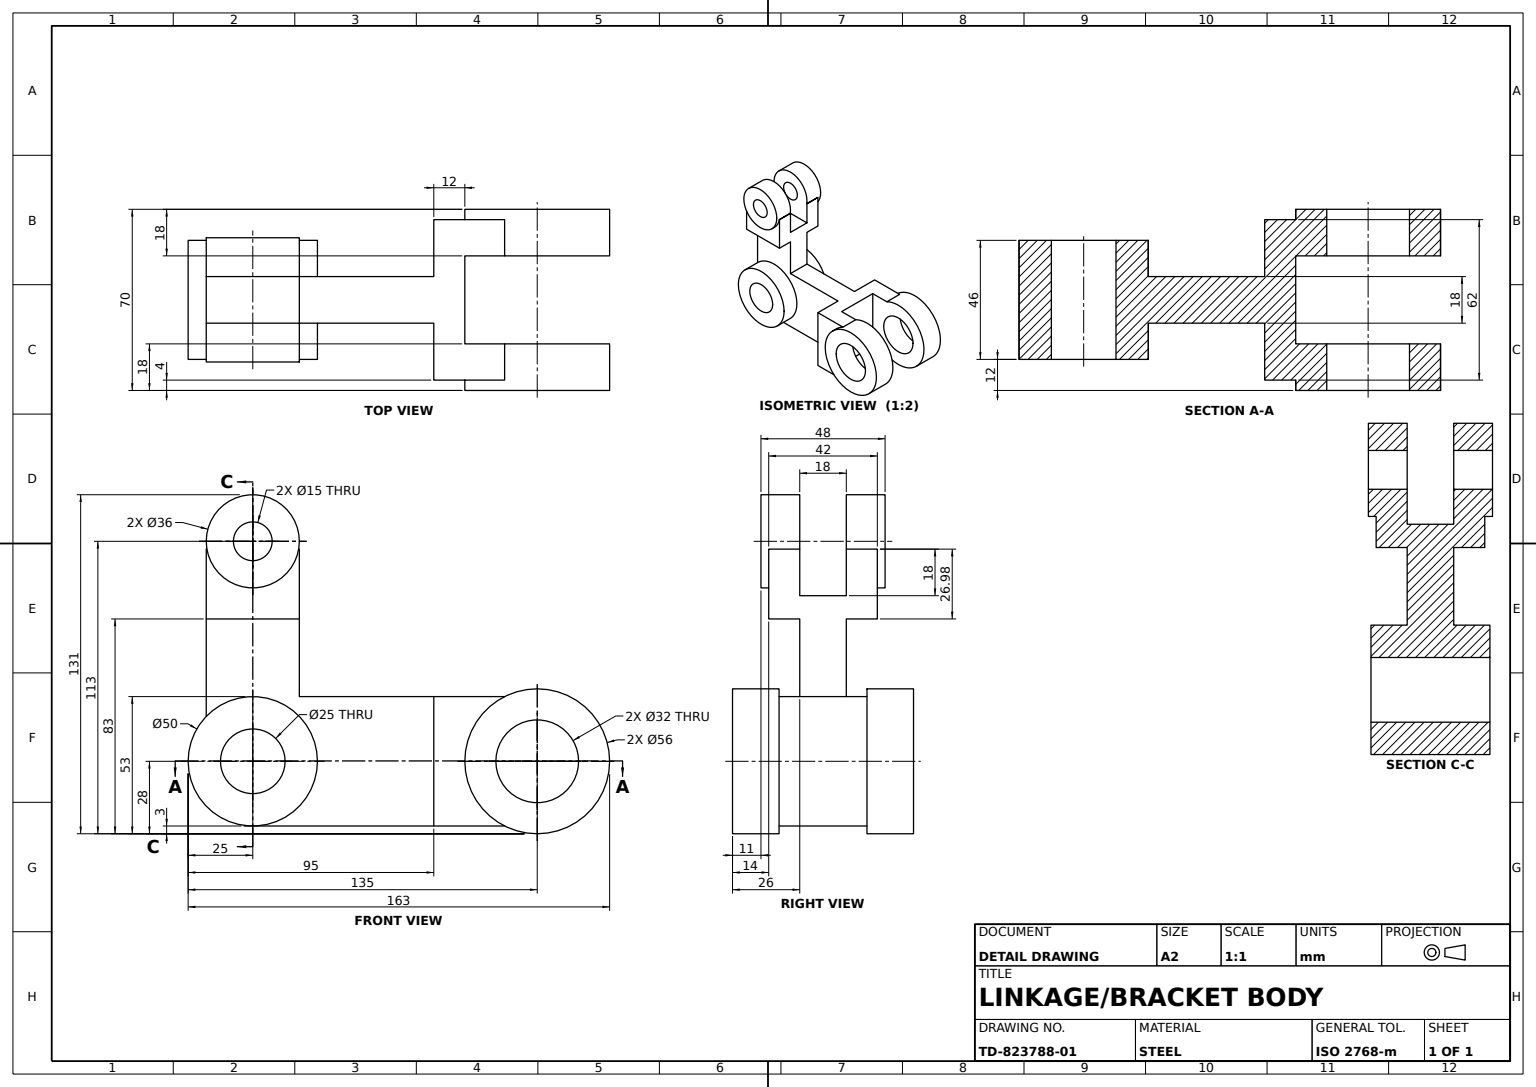
ISO-10303-21;
HEADER;
FILE_DESCRIPTION((''),'2;1');
FILE_NAME('','',(''),(''),'','','');
FILE_SCHEMA(('AUTOMOTIVE_DESIGN'));
ENDSEC;
DATA;
#1=APPLICATION_CONTEXT('');
#2=PRODUCT_CONTEXT('',#1,'mechanical');
#3=PRODUCT('','','',(#2));
#4=PRODUCT_DEFINITION_FORMATION('','',#3);
#5=PRODUCT_DEFINITION_CONTEXT('',#1,'design');
#6=PRODUCT_DEFINITION('','',#4,#5);
#7=PRODUCT_DEFINITION_SHAPE('','',#6);
#8=(LENGTH_UNIT()NAMED_UNIT(*)SI_UNIT(.MILLI.,.METRE.));
#9=(NAMED_UNIT(*)PLANE_ANGLE_UNIT()SI_UNIT($,.RADIAN.));
#10=(NAMED_UNIT(*)SI_UNIT($,.STERADIAN.)SOLID_ANGLE_UNIT());
#11=UNCERTAINTY_MEASURE_WITH_UNIT(LENGTH_MEASURE(1.E-05),#8,'distance_accuracy_value','');
#12=(GEOMETRIC_REPRESENTATION_CONTEXT(3)GLOBAL_UNCERTAINTY_ASSIGNED_CONTEXT((#11))GLOBAL_UNIT_ASSIGNED_CONTEXT((#8,#9,#10))REPRESENTATION_CONTEXT('',''));
#13=CARTESIAN_POINT('',(7.,110.,89.5));
#14=VERTEX_POINT('',#13);
#15=CARTESIAN_POINT('',(22.,110.,89.5));
#16=VERTEX_POINT('',#15);
#17=CARTESIAN_POINT('',(-5.,110.,89.5));
#18=DIRECTION('',(1.,0.,0.));
#19=VECTOR('',#18,1000.);
#20=LINE('',#17,#19);
#21=EDGE_CURVE('',#14,#16,#20,.T.);
#22=ORIENTED_EDGE('',*,*,#21,.F.);
#23=CARTESIAN_POINT('',(7.,110.,74.5));
#24=VERTEX_POINT('',#23);
#25=CARTESIAN_POINT('',(7.,110.,82.));
#26=DIRECTION('',(-1.,0.,0.));
#27=DIRECTION('',(0.,0.,1.));
#28=AXIS2_PLACEMENT_3D('',#25,#26,#27);
#29=CIRCLE('',#28,7.5);
#30=EDGE_CURVE('',#14,#24,#29,.T.);
#31=ORIENTED_EDGE('',*,*,#30,.T.);
#32=CARTESIAN_POINT('',(22.,110.,74.5));
#33=VERTEX_POINT('',#32);
#34=CARTESIAN_POINT('',(-5.,110.,74.5));
#35=LINE('',#34,#19);
#36=EDGE_CURVE('',#24,#33,#35,.T.);
#37=ORIENTED_EDGE('',*,*,#36,.T.);
#38=CARTESIAN_POINT('',(22.,110.,82.));
#39=AXIS2_PLACEMENT_3D('',#38,#26,#27);
#40=CIRCLE('',#39,7.5);
#41=EDGE_CURVE('',#16,#33,#40,.T.);
#42=ORIENTED_EDGE('',*,*,#41,.F.);
#43=EDGE_LOOP('',(#22,#31,#37,#42));
#44=FACE_OUTER_BOUND('',#43,.T.);
#45=CARTESIAN_POINT('',(-5.,110.,82.));
#46=DIRECTION('',(0.,0.,-1.));
#47=AXIS2_PLACEMENT_3D('',#45,#18,#46);
#48=CYLINDRICAL_SURFACE('',#47,7.5);
#49=ADVANCED_FACE('',(#44),#48,.F.);
#50=CARTESIAN_POINT('',(66.,25.,0.));
#51=VERTEX_POINT('',#50);
#52=CARTESIAN_POINT('',(66.,25.,-56.));
#53=VERTEX_POINT('',#52);
#54=CARTESIAN_POINT('',(66.,25.,-28.));
#55=AXIS2_PLACEMENT_3D('',#54,#18,#46);
#56=CIRCLE('',#55,28.);
#57=EDGE_CURVE('',#51,#53,#56,.T.);
#58=ORIENTED_EDGE('',*,*,#57,.T.);
#59=EDGE_CURVE('',#53,#51,#56,.T.);
#60=ORIENTED_EDGE('',*,*,#59,.T.);
#61=EDGE_LOOP('',(#58,#60));
#62=FACE_OUTER_BOUND('',#61,.T.);
#63=CARTESIAN_POINT('',(66.,25.,-44.));
#64=VERTEX_POINT('',#63);
#65=CARTESIAN_POINT('',(66.,25.,-12.));
#66=VERTEX_POINT('',#65);
#67=CIRCLE('',#55,16.);
#68=EDGE_CURVE('',#64,#66,#67,.T.);
#69=ORIENTED_EDGE('',*,*,#68,.F.);
#70=EDGE_CURVE('',#66,#64,#67,.T.);
#71=ORIENTED_EDGE('',*,*,#70,.F.);
#72=EDGE_LOOP('',(#69,#71));
#73=FACE_BOUND('',#72,.T.);
#74=PLANE('',#55);
#75=ADVANCED_FACE('',(#62,#73),#74,.T.);
#76=CARTESIAN_POINT('',(22.,80.,64.));
#77=VERTEX_POINT('',#76);
#78=CARTESIAN_POINT('',(10.,80.,64.));
#79=VERTEX_POINT('',#78);
#80=VECTOR('',#26,1000.);
#81=LINE('',#76,#80);
#82=EDGE_CURVE('',#77,#79,#81,.T.);
#83=ORIENTED_EDGE('',*,*,#82,.F.);
#84=CARTESIAN_POINT('',(22.,80.,100.));
#85=VERTEX_POINT('',#84);
#86=VECTOR('',#46,1000.);
#87=LINE('',#76,#86);
#88=EDGE_CURVE('',#85,#77,#87,.T.);
#89=ORIENTED_EDGE('',*,*,#88,.F.);
#90=CARTESIAN_POINT('',(10.,80.,100.));
#91=VERTEX_POINT('',#90);
#92=LINE('',#84,#80);
#93=EDGE_CURVE('',#85,#91,#92,.T.);
#94=ORIENTED_EDGE('',*,*,#93,.T.);
#95=LINE('',#78,#86);
#96=EDGE_CURVE('',#91,#79,#95,.T.);
#97=ORIENTED_EDGE('',*,*,#96,.T.);
#98=EDGE_LOOP('',(#83,#89,#94,#97));
#99=FACE_OUTER_BOUND('',#98,.T.);
#100=DIRECTION('',(0.,1.,0.));
#101=AXIS2_PLACEMENT_3D('',#76,#100,#27);
#102=PLANE('',#101);
#103=ADVANCED_FACE('',(#99),#102,.F.);
#104=CARTESIAN_POINT('',(40.,0.,85.354634));
#105=VERTEX_POINT('',#104);
#106=CARTESIAN_POINT('',(40.,0.226094,85.354634));
#107=VERTEX_POINT('',#106);
#108=VECTOR('',#100,1000.);
#109=LINE('',#104,#108);
#110=EDGE_CURVE('',#105,#107,#109,.T.);
#111=ORIENTED_EDGE('',*,*,#110,.F.);
#112=CARTESIAN_POINT('',(40.,0.,82.));
#113=VERTEX_POINT('',#112);
#114=LINE('',#104,#86);
#115=EDGE_CURVE('',#105,#113,#114,.T.);
#116=ORIENTED_EDGE('',*,*,#115,.T.);
#117=CARTESIAN_POINT('',(40.,25.,82.));
#118=AXIS2_PLACEMENT_3D('',#117,#26,#46);
#119=CIRCLE('',#118,25.);
#120=EDGE_CURVE('',#113,#107,#119,.T.);
#121=ORIENTED_EDGE('',*,*,#120,.T.);
#122=EDGE_LOOP('',(#111,#116,#121));
#123=FACE_OUTER_BOUND('',#122,.T.);
#124=CARTESIAN_POINT('',(40.,0.,71.244384));
#125=AXIS2_PLACEMENT_3D('',#124,#18,#46);
#126=PLANE('',#125);
#127=ADVANCED_FACE('',(#123),#126,.T.);
#128=CARTESIAN_POINT('',(40.,106.982899,100.));
#129=VERTEX_POINT('',#128);
#130=CARTESIAN_POINT('',(52.,106.982899,100.));
#131=VERTEX_POINT('',#130);
#132=CARTESIAN_POINT('',(0.,106.982899,100.));
#133=LINE('',#132,#19);
#134=EDGE_CURVE('',#129,#131,#133,.T.);
#135=ORIENTED_EDGE('',*,*,#134,.F.);
#136=CARTESIAN_POINT('',(40.,88.982899,100.));
#137=VERTEX_POINT('',#136);
#138=CARTESIAN_POINT('',(40.,0.,100.));
#139=LINE('',#138,#108);
#140=EDGE_CURVE('',#137,#129,#139,.T.);
#141=ORIENTED_EDGE('',*,*,#140,.F.);
#142=CARTESIAN_POINT('',(22.,88.982899,100.));
#143=VERTEX_POINT('',#142);
#144=LINE('',#142,#80);
#145=EDGE_CURVE('',#137,#143,#144,.T.);
#146=ORIENTED_EDGE('',*,*,#145,.T.);
#147=CARTESIAN_POINT('',(22.,106.982899,100.));
#148=VERTEX_POINT('',#147);
#149=CARTESIAN_POINT('',(22.,0.,100.));
#150=DIRECTION('',(0.,-1.,0.));
#151=VECTOR('',#150,1000.);
#152=LINE('',#149,#151);
#153=EDGE_CURVE('',#148,#143,#152,.T.);
#154=ORIENTED_EDGE('',*,*,#153,.F.);
#155=CARTESIAN_POINT('',(10.,106.982899,100.));
#156=VERTEX_POINT('',#155);
#157=EDGE_CURVE('',#156,#148,#133,.T.);
#158=ORIENTED_EDGE('',*,*,#157,.F.);
#159=CARTESIAN_POINT('',(10.,0.,100.));
#160=LINE('',#159,#108);
#161=EDGE_CURVE('',#91,#156,#160,.T.);
#162=ORIENTED_EDGE('',*,*,#161,.F.);
#163=ORIENTED_EDGE('',*,*,#93,.F.);
#164=CARTESIAN_POINT('',(22.,42.349352,100.));
#165=VERTEX_POINT('',#164);
#166=EDGE_CURVE('',#85,#165,#152,.T.);
#167=ORIENTED_EDGE('',*,*,#166,.T.);
#168=CARTESIAN_POINT('',(40.,42.349352,100.));
#169=VERTEX_POINT('',#168);
#170=CARTESIAN_POINT('',(0.,42.349352,100.));
#171=LINE('',#170,#19);
#172=EDGE_CURVE('',#165,#169,#171,.T.);
#173=ORIENTED_EDGE('',*,*,#172,.T.);
#174=CARTESIAN_POINT('',(40.,80.,100.));
#175=VERTEX_POINT('',#174);
#176=EDGE_CURVE('',#169,#175,#139,.T.);
#177=ORIENTED_EDGE('',*,*,#176,.T.);
#178=CARTESIAN_POINT('',(52.,80.,100.));
#179=VERTEX_POINT('',#178);
#180=LINE('',#174,#19);
#181=EDGE_CURVE('',#175,#179,#180,.T.);
#182=ORIENTED_EDGE('',*,*,#181,.T.);
#183=CARTESIAN_POINT('',(52.,0.,100.));
#184=LINE('',#183,#151);
#185=EDGE_CURVE('',#131,#179,#184,.T.);
#186=ORIENTED_EDGE('',*,*,#185,.F.);
#187=EDGE_LOOP('',(#135,#141,#146,#154,#158,#162,#163,#167,#173,#177,#182,#186));
#188=FACE_OUTER_BOUND('',#187,.T.);
#189=CARTESIAN_POINT('',(0.,0.,100.));
#190=AXIS2_PLACEMENT_3D('',#189,#27,#18);
#191=PLANE('',#190);
#192=ADVANCED_FACE('',(#188),#191,.T.);
#193=CARTESIAN_POINT('',(22.,106.982899,99.74534));
#194=VERTEX_POINT('',#193);
#195=CARTESIAN_POINT('',(22.,106.982899,64.));
#196=VECTOR('',#27,1000.);
#197=LINE('',#195,#196);
#198=EDGE_CURVE('',#194,#148,#197,.T.);
#199=ORIENTED_EDGE('',*,*,#198,.F.);
#200=CARTESIAN_POINT('',(10.,106.982899,99.74534));
#201=VERTEX_POINT('',#200);
#202=CARTESIAN_POINT('',(7.,106.982899,99.74534));
#203=LINE('',#202,#19);
#204=EDGE_CURVE('',#201,#194,#203,.T.);
#205=ORIENTED_EDGE('',*,*,#204,.F.);
#206=CARTESIAN_POINT('',(10.,106.982899,64.));
#207=LINE('',#206,#196);
#208=EDGE_CURVE('',#201,#156,#207,.T.);
#209=ORIENTED_EDGE('',*,*,#208,.T.);
#210=ORIENTED_EDGE('',*,*,#157,.T.);
#211=EDGE_LOOP('',(#199,#205,#209,#210));
#212=FACE_OUTER_BOUND('',#211,.T.);
#213=CARTESIAN_POINT('',(0.,106.982899,64.));
#214=AXIS2_PLACEMENT_3D('',#213,#150,#46);
#215=PLANE('',#214);
#216=ADVANCED_FACE('',(#212),#215,.F.);
#217=CARTESIAN_POINT('',(22.,0.,12.));
#218=VERTEX_POINT('',#217);
#219=CARTESIAN_POINT('',(22.,50.,12.));
#220=VERTEX_POINT('',#219);
#221=LINE('',#217,#108);
#222=EDGE_CURVE('',#218,#220,#221,.T.);
#223=ORIENTED_EDGE('',*,*,#222,.T.);
#224=CARTESIAN_POINT('',(0.,50.,12.));
#225=VERTEX_POINT('',#224);
#226=LINE('',#224,#80);
#227=EDGE_CURVE('',#220,#225,#226,.T.);
#228=ORIENTED_EDGE('',*,*,#227,.T.);
#229=CARTESIAN_POINT('',(0.,0.,12.));
#230=VERTEX_POINT('',#229);
#231=LINE('',#229,#151);
#232=EDGE_CURVE('',#225,#230,#231,.T.);
#233=ORIENTED_EDGE('',*,*,#232,.T.);
#234=LINE('',#229,#19);
#235=EDGE_CURVE('',#230,#218,#234,.T.);
#236=ORIENTED_EDGE('',*,*,#235,.T.);
#237=EDGE_LOOP('',(#223,#228,#233,#236));
#238=FACE_OUTER_BOUND('',#237,.T.);
#239=AXIS2_PLACEMENT_3D('',#229,#46,#26);
#240=PLANE('',#239);
#241=ADVANCED_FACE('',(#238),#240,.F.);
#242=CARTESIAN_POINT('',(14.,0.,-15.39048));
#243=VERTEX_POINT('',#242);
#244=CARTESIAN_POINT('',(0.,0.,-15.39048));
#245=VERTEX_POINT('',#244);
#246=LINE('',#242,#80);
#247=EDGE_CURVE('',#243,#245,#246,.T.);
#248=ORIENTED_EDGE('',*,*,#247,.T.);
#249=CARTESIAN_POINT('',(0.,25.,0.));
#250=VERTEX_POINT('',#249);
#251=CARTESIAN_POINT('',(0.,25.,-28.));
#252=AXIS2_PLACEMENT_3D('',#251,#26,#27);
#253=CIRCLE('',#252,28.);
#254=EDGE_CURVE('',#245,#250,#253,.T.);
#255=ORIENTED_EDGE('',*,*,#254,.T.);
#256=CARTESIAN_POINT('',(-4.,25.,0.));
#257=VERTEX_POINT('',#256);
#258=CARTESIAN_POINT('',(14.,25.,0.));
#259=LINE('',#258,#80);
#260=EDGE_CURVE('',#250,#257,#259,.T.);
#261=ORIENTED_EDGE('',*,*,#260,.T.);
#262=CARTESIAN_POINT('',(-4.,25.,-56.));
#263=VERTEX_POINT('',#262);
#264=CARTESIAN_POINT('',(-4.,25.,-28.));
#265=AXIS2_PLACEMENT_3D('',#264,#26,#27);
#266=CIRCLE('',#265,28.);
#267=EDGE_CURVE('',#263,#257,#266,.T.);
#268=ORIENTED_EDGE('',*,*,#267,.F.);
#269=CARTESIAN_POINT('',(14.,25.,-56.));
#270=VERTEX_POINT('',#269);
#271=LINE('',#269,#80);
#272=EDGE_CURVE('',#270,#263,#271,.T.);
#273=ORIENTED_EDGE('',*,*,#272,.F.);
#274=CARTESIAN_POINT('',(14.,25.,-28.));
#275=AXIS2_PLACEMENT_3D('',#274,#26,#27);
#276=CIRCLE('',#275,28.);
#277=EDGE_CURVE('',#270,#243,#276,.T.);
#278=ORIENTED_EDGE('',*,*,#277,.T.);
#279=EDGE_LOOP('',(#248,#255,#261,#268,#273,#278));
#280=FACE_OUTER_BOUND('',#279,.T.);
#281=CYLINDRICAL_SURFACE('',#275,28.);
#282=ADVANCED_FACE('',(#280),#281,.T.);
#283=CARTESIAN_POINT('',(52.,106.982899,64.25466));
#284=VERTEX_POINT('',#283);
#285=CARTESIAN_POINT('',(40.,106.982899,64.25466));
#286=VERTEX_POINT('',#285);
#287=CARTESIAN_POINT('',(55.,106.982899,64.25466));
#288=LINE('',#287,#80);
#289=EDGE_CURVE('',#284,#286,#288,.T.);
#290=ORIENTED_EDGE('',*,*,#289,.F.);
#291=CARTESIAN_POINT('',(52.,106.982899,64.));
#292=VERTEX_POINT('',#291);
#293=LINE('',#291,#196);
#294=EDGE_CURVE('',#292,#284,#293,.T.);
#295=ORIENTED_EDGE('',*,*,#294,.F.);
#296=CARTESIAN_POINT('',(40.,106.982899,64.));
#297=VERTEX_POINT('',#296);
#298=LINE('',#213,#19);
#299=EDGE_CURVE('',#297,#292,#298,.T.);
#300=ORIENTED_EDGE('',*,*,#299,.F.);
#301=LINE('',#296,#196);
#302=EDGE_CURVE('',#297,#286,#301,.T.);
#303=ORIENTED_EDGE('',*,*,#302,.T.);
#304=EDGE_LOOP('',(#290,#295,#300,#303));
#305=FACE_OUTER_BOUND('',#304,.T.);
#306=ADVANCED_FACE('',(#305),#215,.F.);
#307=CARTESIAN_POINT('',(48.,25.,-12.));
#308=VERTEX_POINT('',#307);
#309=CARTESIAN_POINT('',(-14.,25.,-12.));
#310=LINE('',#309,#19);
#311=EDGE_CURVE('',#308,#66,#310,.T.);
#312=ORIENTED_EDGE('',*,*,#311,.T.);
#313=ORIENTED_EDGE('',*,*,#70,.T.);
#314=CARTESIAN_POINT('',(48.,25.,-44.));
#315=VERTEX_POINT('',#314);
#316=CARTESIAN_POINT('',(-14.,25.,-44.));
#317=LINE('',#316,#19);
#318=EDGE_CURVE('',#315,#64,#317,.T.);
#319=ORIENTED_EDGE('',*,*,#318,.F.);
#320=CARTESIAN_POINT('',(48.,25.,-28.));
#321=AXIS2_PLACEMENT_3D('',#320,#18,#46);
#322=CIRCLE('',#321,16.);
#323=EDGE_CURVE('',#308,#315,#322,.T.);
#324=ORIENTED_EDGE('',*,*,#323,.F.);
#325=EDGE_LOOP('',(#312,#313,#319,#324));
#326=FACE_OUTER_BOUND('',#325,.T.);
#327=CARTESIAN_POINT('',(-14.,25.,-28.));
#328=AXIS2_PLACEMENT_3D('',#327,#18,#46);
#329=CYLINDRICAL_SURFACE('',#328,16.);
#330=ADVANCED_FACE('',(#326),#329,.F.);
#331=CARTESIAN_POINT('',(62.,50.,12.));
#332=VERTEX_POINT('',#331);
#333=CARTESIAN_POINT('',(40.,50.,12.));
#334=VERTEX_POINT('',#333);
#335=EDGE_CURVE('',#332,#334,#226,.T.);
#336=ORIENTED_EDGE('',*,*,#335,.T.);
#337=CARTESIAN_POINT('',(40.,0.,12.));
#338=VERTEX_POINT('',#337);
#339=LINE('',#337,#108);
#340=EDGE_CURVE('',#338,#334,#339,.T.);
#341=ORIENTED_EDGE('',*,*,#340,.F.);
#342=CARTESIAN_POINT('',(62.,0.,12.));
#343=VERTEX_POINT('',#342);
#344=EDGE_CURVE('',#338,#343,#234,.T.);
#345=ORIENTED_EDGE('',*,*,#344,.T.);
#346=LINE('',#331,#108);
#347=EDGE_CURVE('',#343,#332,#346,.T.);
#348=ORIENTED_EDGE('',*,*,#347,.T.);
#349=EDGE_LOOP('',(#336,#341,#345,#348));
#350=FACE_OUTER_BOUND('',#349,.T.);
#351=ADVANCED_FACE('',(#350),#240,.F.);
#352=EDGE_CURVE('',#24,#14,#29,.T.);
#353=ORIENTED_EDGE('',*,*,#352,.T.);
#354=ORIENTED_EDGE('',*,*,#21,.T.);
#355=EDGE_CURVE('',#33,#16,#40,.T.);
#356=ORIENTED_EDGE('',*,*,#355,.F.);
#357=ORIENTED_EDGE('',*,*,#36,.F.);
#358=EDGE_LOOP('',(#353,#354,#356,#357));
#359=FACE_OUTER_BOUND('',#358,.T.);
#360=ADVANCED_FACE('',(#359),#48,.F.);
#361=CARTESIAN_POINT('',(55.,110.,89.5));
#362=VERTEX_POINT('',#361);
#363=CARTESIAN_POINT('',(55.,110.,74.5));
#364=VERTEX_POINT('',#363);
#365=CARTESIAN_POINT('',(55.,110.,82.));
#366=AXIS2_PLACEMENT_3D('',#365,#18,#46);
#367=CIRCLE('',#366,7.5);
#368=EDGE_CURVE('',#362,#364,#367,.T.);
#369=ORIENTED_EDGE('',*,*,#368,.F.);
#370=EDGE_CURVE('',#364,#362,#367,.T.);
#371=ORIENTED_EDGE('',*,*,#370,.F.);
#372=EDGE_LOOP('',(#369,#371));
#373=FACE_BOUND('',#372,.T.);
#374=CARTESIAN_POINT('',(55.,110.,100.));
#375=VERTEX_POINT('',#374);
#376=CARTESIAN_POINT('',(55.,110.,64.));
#377=VERTEX_POINT('',#376);
#378=CIRCLE('',#366,18.);
#379=EDGE_CURVE('',#375,#377,#378,.T.);
#380=ORIENTED_EDGE('',*,*,#379,.T.);
#381=EDGE_CURVE('',#377,#375,#378,.T.);
#382=ORIENTED_EDGE('',*,*,#381,.T.);
#383=EDGE_LOOP('',(#380,#382));
#384=FACE_OUTER_BOUND('',#383,.T.);
#385=PLANE('',#366);
#386=ADVANCED_FACE('',(#373,#384),#385,.T.);
#387=CARTESIAN_POINT('',(62.,25.,0.));
#388=VERTEX_POINT('',#387);
#389=CARTESIAN_POINT('',(62.,0.,-15.39048));
#390=VERTEX_POINT('',#389);
#391=CARTESIAN_POINT('',(62.,25.,-28.));
#392=AXIS2_PLACEMENT_3D('',#391,#18,#46);
#393=CIRCLE('',#392,28.);
#394=EDGE_CURVE('',#388,#390,#393,.T.);
#395=ORIENTED_EDGE('',*,*,#394,.F.);
#396=CARTESIAN_POINT('',(62.,50.,-15.39048));
#397=VERTEX_POINT('',#396);
#398=EDGE_CURVE('',#397,#388,#393,.T.);
#399=ORIENTED_EDGE('',*,*,#398,.F.);
#400=LINE('',#331,#86);
#401=EDGE_CURVE('',#332,#397,#400,.T.);
#402=ORIENTED_EDGE('',*,*,#401,.F.);
#403=ORIENTED_EDGE('',*,*,#347,.F.);
#404=LINE('',#342,#86);
#405=EDGE_CURVE('',#343,#390,#404,.T.);
#406=ORIENTED_EDGE('',*,*,#405,.T.);
#407=EDGE_LOOP('',(#395,#399,#402,#403,#406));
#408=FACE_OUTER_BOUND('',#407,.T.);
#409=AXIS2_PLACEMENT_3D('',#331,#26,#27);
#410=PLANE('',#409);
#411=ADVANCED_FACE('',(#408),#410,.F.);
#412=CARTESIAN_POINT('',(40.,106.982899,99.74534));
#413=VERTEX_POINT('',#412);
#414=CARTESIAN_POINT('',(52.,106.982899,99.74534));
#415=VERTEX_POINT('',#414);
#416=CARTESIAN_POINT('',(55.,106.982899,99.74534));
#417=LINE('',#416,#19);
#418=EDGE_CURVE('',#413,#415,#417,.T.);
#419=ORIENTED_EDGE('',*,*,#418,.T.);
#420=CARTESIAN_POINT('',(52.,110.,82.));
#421=AXIS2_PLACEMENT_3D('',#420,#18,#27);
#422=CIRCLE('',#421,18.);
#423=EDGE_CURVE('',#415,#284,#422,.T.);
#424=ORIENTED_EDGE('',*,*,#423,.T.);
#425=ORIENTED_EDGE('',*,*,#289,.T.);
#426=CARTESIAN_POINT('',(40.,110.,64.));
#427=VERTEX_POINT('',#426);
#428=CARTESIAN_POINT('',(40.,110.,82.));
#429=AXIS2_PLACEMENT_3D('',#428,#18,#46);
#430=CIRCLE('',#429,18.);
#431=EDGE_CURVE('',#286,#427,#430,.T.);
#432=ORIENTED_EDGE('',*,*,#431,.T.);
#433=LINE('',#376,#80);
#434=EDGE_CURVE('',#377,#427,#433,.T.);
#435=ORIENTED_EDGE('',*,*,#434,.F.);
#436=ORIENTED_EDGE('',*,*,#379,.F.);
#437=CARTESIAN_POINT('',(40.,110.,100.));
#438=VERTEX_POINT('',#437);
#439=LINE('',#374,#80);
#440=EDGE_CURVE('',#375,#438,#439,.T.);
#441=ORIENTED_EDGE('',*,*,#440,.T.);
#442=EDGE_CURVE('',#438,#413,#430,.T.);
#443=ORIENTED_EDGE('',*,*,#442,.T.);
#444=EDGE_LOOP('',(#419,#424,#425,#432,#435,#436,#441,#443));
#445=FACE_OUTER_BOUND('',#444,.T.);
#446=AXIS2_PLACEMENT_3D('',#365,#26,#27);
#447=CYLINDRICAL_SURFACE('',#446,18.);
#448=ADVANCED_FACE('',(#445),#447,.T.);
#449=CARTESIAN_POINT('',(7.,110.,64.));
#450=VERTEX_POINT('',#449);
#451=CARTESIAN_POINT('',(22.,110.,64.));
#452=VERTEX_POINT('',#451);
#453=LINE('',#449,#19);
#454=EDGE_CURVE('',#450,#452,#453,.T.);
#455=ORIENTED_EDGE('',*,*,#454,.F.);
#456=CARTESIAN_POINT('',(7.,110.,100.));
#457=VERTEX_POINT('',#456);
#458=CIRCLE('',#28,18.);
#459=EDGE_CURVE('',#457,#450,#458,.T.);
#460=ORIENTED_EDGE('',*,*,#459,.F.);
#461=CARTESIAN_POINT('',(22.,110.,100.));
#462=VERTEX_POINT('',#461);
#463=LINE('',#456,#19);
#464=EDGE_CURVE('',#457,#462,#463,.T.);
#465=ORIENTED_EDGE('',*,*,#464,.T.);
#466=CIRCLE('',#39,18.);
#467=EDGE_CURVE('',#462,#452,#466,.T.);
#468=ORIENTED_EDGE('',*,*,#467,.T.);
#469=EDGE_LOOP('',(#455,#460,#465,#468));
#470=FACE_OUTER_BOUND('',#469,.T.);
#471=AXIS2_PLACEMENT_3D('',#25,#18,#46);
#472=CYLINDRICAL_SURFACE('',#471,18.);
#473=ADVANCED_FACE('',(#470),#472,.T.);
#474=CARTESIAN_POINT('',(-4.,25.,-12.));
#475=VERTEX_POINT('',#474);
#476=CARTESIAN_POINT('',(14.,25.,-12.));
#477=VERTEX_POINT('',#476);
#478=EDGE_CURVE('',#475,#477,#310,.T.);
#479=ORIENTED_EDGE('',*,*,#478,.F.);
#480=CARTESIAN_POINT('',(-4.,25.,-44.));
#481=VERTEX_POINT('',#480);
#482=CIRCLE('',#265,16.);
#483=EDGE_CURVE('',#475,#481,#482,.T.);
#484=ORIENTED_EDGE('',*,*,#483,.T.);
#485=CARTESIAN_POINT('',(14.,25.,-44.));
#486=VERTEX_POINT('',#485);
#487=EDGE_CURVE('',#481,#486,#317,.T.);
#488=ORIENTED_EDGE('',*,*,#487,.T.);
#489=CIRCLE('',#275,16.);
#490=EDGE_CURVE('',#477,#486,#489,.T.);
#491=ORIENTED_EDGE('',*,*,#490,.F.);
#492=EDGE_LOOP('',(#479,#484,#488,#491));
#493=FACE_OUTER_BOUND('',#492,.T.);
#494=ADVANCED_FACE('',(#493),#329,.F.);
#495=CARTESIAN_POINT('',(40.,88.982899,64.));
#496=VERTEX_POINT('',#495);
#497=LINE('',#495,#196);
#498=EDGE_CURVE('',#496,#137,#497,.T.);
#499=ORIENTED_EDGE('',*,*,#498,.F.);
#500=CARTESIAN_POINT('',(22.,88.982899,64.));
#501=VERTEX_POINT('',#500);
#502=LINE('',#500,#80);
#503=EDGE_CURVE('',#496,#501,#502,.T.);
#504=ORIENTED_EDGE('',*,*,#503,.T.);
#505=LINE('',#500,#196);
#506=EDGE_CURVE('',#501,#143,#505,.T.);
#507=ORIENTED_EDGE('',*,*,#506,.T.);
#508=ORIENTED_EDGE('',*,*,#145,.F.);
#509=EDGE_LOOP('',(#499,#504,#507,#508));
#510=FACE_OUTER_BOUND('',#509,.T.);
#511=AXIS2_PLACEMENT_3D('',#500,#100,#27);
#512=PLANE('',#511);
#513=ADVANCED_FACE('',(#510),#512,.T.);
#514=CARTESIAN_POINT('',(54.,25.,94.5));
#515=VERTEX_POINT('',#514);
#516=CARTESIAN_POINT('',(8.,25.,94.5));
#517=VERTEX_POINT('',#516);
#518=LINE('',#514,#80);
#519=EDGE_CURVE('',#515,#517,#518,.T.);
#520=ORIENTED_EDGE('',*,*,#519,.T.);
#521=CARTESIAN_POINT('',(8.,25.,69.5));
#522=VERTEX_POINT('',#521);
#523=CARTESIAN_POINT('',(8.,25.,82.));
#524=AXIS2_PLACEMENT_3D('',#523,#26,#27);
#525=CIRCLE('',#524,12.5);
#526=EDGE_CURVE('',#517,#522,#525,.T.);
#527=ORIENTED_EDGE('',*,*,#526,.T.);
#528=CARTESIAN_POINT('',(54.,25.,69.5));
#529=VERTEX_POINT('',#528);
#530=LINE('',#528,#80);
#531=EDGE_CURVE('',#529,#522,#530,.T.);
#532=ORIENTED_EDGE('',*,*,#531,.F.);
#533=CARTESIAN_POINT('',(54.,25.,82.));
#534=AXIS2_PLACEMENT_3D('',#533,#26,#27);
#535=CIRCLE('',#534,12.5);
#536=EDGE_CURVE('',#515,#529,#535,.T.);
#537=ORIENTED_EDGE('',*,*,#536,.F.);
#538=EDGE_LOOP('',(#520,#527,#532,#537));
#539=FACE_OUTER_BOUND('',#538,.T.);
#540=CYLINDRICAL_SURFACE('',#534,12.5);
#541=ADVANCED_FACE('',(#539),#540,.F.);
#542=ORIENTED_EDGE('',*,*,#352,.F.);
#543=ORIENTED_EDGE('',*,*,#30,.F.);
#544=EDGE_LOOP('',(#542,#543));
#545=FACE_BOUND('',#544,.T.);
#546=EDGE_CURVE('',#450,#457,#458,.T.);
#547=ORIENTED_EDGE('',*,*,#546,.T.);
#548=ORIENTED_EDGE('',*,*,#459,.T.);
#549=EDGE_LOOP('',(#547,#548));
#550=FACE_OUTER_BOUND('',#549,.T.);
#551=CARTESIAN_POINT('',(7.,0.,0.));
#552=AXIS2_PLACEMENT_3D('',#551,#26,#27);
#553=PLANE('',#552);
#554=ADVANCED_FACE('',(#545,#550),#553,.T.);
#555=CARTESIAN_POINT('',(14.,50.,-15.39048));
#556=VERTEX_POINT('',#555);
#557=EDGE_CURVE('',#556,#270,#276,.T.);
#558=ORIENTED_EDGE('',*,*,#557,.T.);
#559=ORIENTED_EDGE('',*,*,#272,.T.);
#560=EDGE_CURVE('',#257,#263,#266,.T.);
#561=ORIENTED_EDGE('',*,*,#560,.F.);
#562=ORIENTED_EDGE('',*,*,#260,.F.);
#563=CARTESIAN_POINT('',(0.,50.,-15.39048));
#564=VERTEX_POINT('',#563);
#565=EDGE_CURVE('',#250,#564,#253,.T.);
#566=ORIENTED_EDGE('',*,*,#565,.T.);
#567=LINE('',#555,#80);
#568=EDGE_CURVE('',#556,#564,#567,.T.);
#569=ORIENTED_EDGE('',*,*,#568,.F.);
#570=EDGE_LOOP('',(#558,#559,#561,#562,#566,#569));
#571=FACE_OUTER_BOUND('',#570,.T.);
#572=ADVANCED_FACE('',(#571),#281,.T.);
#573=EDGE_CURVE('',#522,#517,#525,.T.);
#574=ORIENTED_EDGE('',*,*,#573,.T.);
#575=ORIENTED_EDGE('',*,*,#519,.F.);
#576=EDGE_CURVE('',#529,#515,#535,.T.);
#577=ORIENTED_EDGE('',*,*,#576,.F.);
#578=ORIENTED_EDGE('',*,*,#531,.T.);
#579=EDGE_LOOP('',(#574,#575,#577,#578));
#580=FACE_OUTER_BOUND('',#579,.T.);
#581=ADVANCED_FACE('',(#580),#540,.F.);
#582=CARTESIAN_POINT('',(40.,110.,89.5));
#583=VERTEX_POINT('',#582);
#584=CARTESIAN_POINT('',(40.,110.,74.5));
#585=VERTEX_POINT('',#584);
#586=CIRCLE('',#429,7.5);
#587=EDGE_CURVE('',#583,#585,#586,.T.);
#588=ORIENTED_EDGE('',*,*,#587,.F.);
#589=EDGE_CURVE('',#583,#362,#20,.T.);
#590=ORIENTED_EDGE('',*,*,#589,.T.);
#591=ORIENTED_EDGE('',*,*,#368,.T.);
#592=EDGE_CURVE('',#585,#364,#35,.T.);
#593=ORIENTED_EDGE('',*,*,#592,.F.);
#594=EDGE_LOOP('',(#588,#590,#591,#593));
#595=FACE_OUTER_BOUND('',#594,.T.);
#596=ADVANCED_FACE('',(#595),#48,.F.);
#597=ORIENTED_EDGE('',*,*,#589,.F.);
#598=EDGE_CURVE('',#585,#583,#586,.T.);
#599=ORIENTED_EDGE('',*,*,#598,.F.);
#600=ORIENTED_EDGE('',*,*,#592,.T.);
#601=ORIENTED_EDGE('',*,*,#370,.T.);
#602=EDGE_LOOP('',(#597,#599,#600,#601));
#603=FACE_OUTER_BOUND('',#602,.T.);
#604=ADVANCED_FACE('',(#603),#48,.F.);
#605=CARTESIAN_POINT('',(22.,0.,85.354634));
#606=VERTEX_POINT('',#605);
#607=CARTESIAN_POINT('',(22.,0.226094,85.354634));
#608=VERTEX_POINT('',#607);
#609=LINE('',#605,#108);
#610=EDGE_CURVE('',#606,#608,#609,.T.);
#611=ORIENTED_EDGE('',*,*,#610,.T.);
#612=CARTESIAN_POINT('',(22.,0.,82.));
#613=VERTEX_POINT('',#612);
#614=CARTESIAN_POINT('',(22.,25.,82.));
#615=AXIS2_PLACEMENT_3D('',#614,#18,#27);
#616=CIRCLE('',#615,25.);
#617=EDGE_CURVE('',#608,#613,#616,.T.);
#618=ORIENTED_EDGE('',*,*,#617,.T.);
#619=LINE('',#217,#196);
#620=EDGE_CURVE('',#613,#606,#619,.T.);
#621=ORIENTED_EDGE('',*,*,#620,.T.);
#622=EDGE_LOOP('',(#611,#618,#621));
#623=FACE_OUTER_BOUND('',#622,.T.);
#624=CARTESIAN_POINT('',(22.,0.,71.244384));
#625=AXIS2_PLACEMENT_3D('',#624,#26,#27);
#626=PLANE('',#625);
#627=ADVANCED_FACE('',(#623),#626,.T.);
#628=CARTESIAN_POINT('',(54.,25.,107.));
#629=VERTEX_POINT('',#628);
#630=CARTESIAN_POINT('',(54.,25.,57.));
#631=VERTEX_POINT('',#630);
#632=AXIS2_PLACEMENT_3D('',#533,#18,#46);
#633=CIRCLE('',#632,25.);
#634=EDGE_CURVE('',#629,#631,#633,.T.);
#635=ORIENTED_EDGE('',*,*,#634,.T.);
#636=EDGE_CURVE('',#631,#629,#633,.T.);
#637=ORIENTED_EDGE('',*,*,#636,.T.);
#638=EDGE_LOOP('',(#635,#637));
#639=FACE_OUTER_BOUND('',#638,.T.);
#640=ORIENTED_EDGE('',*,*,#576,.T.);
#641=ORIENTED_EDGE('',*,*,#536,.T.);
#642=EDGE_LOOP('',(#640,#641));
#643=FACE_BOUND('',#642,.T.);
#644=PLANE('',#632);
#645=ADVANCED_FACE('',(#639,#643),#644,.T.);
#646=CARTESIAN_POINT('',(40.,25.,57.));
#647=VERTEX_POINT('',#646);
#648=EDGE_CURVE('',#169,#647,#119,.T.);
#649=ORIENTED_EDGE('',*,*,#648,.T.);
#650=EDGE_CURVE('',#647,#113,#119,.T.);
#651=ORIENTED_EDGE('',*,*,#650,.T.);
#652=EDGE_CURVE('',#113,#338,#114,.T.);
#653=ORIENTED_EDGE('',*,*,#652,.T.);
#654=ORIENTED_EDGE('',*,*,#340,.T.);
#655=CARTESIAN_POINT('',(40.,50.,64.));
#656=VERTEX_POINT('',#655);
#657=CARTESIAN_POINT('',(40.,50.,71.244384));
#658=LINE('',#657,#86);
#659=EDGE_CURVE('',#656,#334,#658,.T.);
#660=ORIENTED_EDGE('',*,*,#659,.F.);
#661=CARTESIAN_POINT('',(40.,80.,64.));
#662=VERTEX_POINT('',#661);
#663=CARTESIAN_POINT('',(40.,0.,64.));
#664=LINE('',#663,#108);
#665=EDGE_CURVE('',#656,#662,#664,.T.);
#666=ORIENTED_EDGE('',*,*,#665,.T.);
#667=LINE('',#174,#196);
#668=EDGE_CURVE('',#662,#175,#667,.T.);
#669=ORIENTED_EDGE('',*,*,#668,.T.);
#670=ORIENTED_EDGE('',*,*,#176,.F.);
#671=EDGE_LOOP('',(#649,#651,#653,#654,#660,#666,#669,#670));
#672=FACE_OUTER_BOUND('',#671,.T.);
#673=ADVANCED_FACE('',(#672),#126,.T.);
#674=ORIENTED_EDGE('',*,*,#355,.T.);
#675=ORIENTED_EDGE('',*,*,#41,.T.);
#676=EDGE_LOOP('',(#674,#675));
#677=FACE_BOUND('',#676,.T.);
#678=ORIENTED_EDGE('',*,*,#506,.F.);
#679=VERTEX_POINT('',#195);
#680=CARTESIAN_POINT('',(22.,0.,64.));
#681=LINE('',#680,#151);
#682=EDGE_CURVE('',#679,#501,#681,.T.);
#683=ORIENTED_EDGE('',*,*,#682,.F.);
#684=CARTESIAN_POINT('',(22.,106.982899,64.25466));
#685=VERTEX_POINT('',#684);
#686=EDGE_CURVE('',#679,#685,#197,.T.);
#687=ORIENTED_EDGE('',*,*,#686,.T.);
#688=EDGE_CURVE('',#452,#685,#466,.T.);
#689=ORIENTED_EDGE('',*,*,#688,.F.);
#690=ORIENTED_EDGE('',*,*,#467,.F.);
#691=EDGE_CURVE('',#194,#462,#466,.T.);
#692=ORIENTED_EDGE('',*,*,#691,.F.);
#693=ORIENTED_EDGE('',*,*,#198,.T.);
#694=ORIENTED_EDGE('',*,*,#153,.T.);
#695=EDGE_LOOP('',(#678,#683,#687,#689,#690,#692,#693,#694));
#696=FACE_OUTER_BOUND('',#695,.T.);
#697=AXIS2_PLACEMENT_3D('',#680,#26,#27);
#698=PLANE('',#697);
#699=ADVANCED_FACE('',(#677,#696),#698,.F.);
#700=ORIENTED_EDGE('',*,*,#110,.T.);
#701=CARTESIAN_POINT('',(0.,0.226094,85.354634));
#702=LINE('',#701,#80);
#703=EDGE_CURVE('',#107,#608,#702,.T.);
#704=ORIENTED_EDGE('',*,*,#703,.T.);
#705=ORIENTED_EDGE('',*,*,#610,.F.);
#706=LINE('',#605,#19);
#707=EDGE_CURVE('',#606,#105,#706,.T.);
#708=ORIENTED_EDGE('',*,*,#707,.T.);
#709=EDGE_LOOP('',(#700,#704,#705,#708));
#710=FACE_OUTER_BOUND('',#709,.T.);
#711=AXIS2_PLACEMENT_3D('',#605,#27,#18);
#712=PLANE('',#711);
#713=ADVANCED_FACE('',(#710),#712,.T.);
#714=ORIENTED_EDGE('',*,*,#161,.T.);
#715=ORIENTED_EDGE('',*,*,#208,.F.);
#716=CARTESIAN_POINT('',(10.,106.982899,64.25466));
#717=VERTEX_POINT('',#716);
#718=CARTESIAN_POINT('',(10.,110.,82.));
#719=AXIS2_PLACEMENT_3D('',#718,#26,#46);
#720=CIRCLE('',#719,18.);
#721=EDGE_CURVE('',#717,#201,#720,.T.);
#722=ORIENTED_EDGE('',*,*,#721,.F.);
#723=VERTEX_POINT('',#206);
#724=EDGE_CURVE('',#723,#717,#207,.T.);
#725=ORIENTED_EDGE('',*,*,#724,.F.);
#726=CARTESIAN_POINT('',(10.,0.,64.));
#727=LINE('',#726,#108);
#728=EDGE_CURVE('',#79,#723,#727,.T.);
#729=ORIENTED_EDGE('',*,*,#728,.F.);
#730=ORIENTED_EDGE('',*,*,#96,.F.);
#731=EDGE_LOOP('',(#714,#715,#722,#725,#729,#730));
#732=FACE_OUTER_BOUND('',#731,.T.);
#733=AXIS2_PLACEMENT_3D('',#726,#18,#46);
#734=PLANE('',#733);
#735=ADVANCED_FACE('',(#732),#734,.F.);
#736=EDGE_CURVE('',#486,#477,#489,.T.);
#737=ORIENTED_EDGE('',*,*,#736,.T.);
#738=ORIENTED_EDGE('',*,*,#490,.T.);
#739=EDGE_LOOP('',(#737,#738));
#740=FACE_BOUND('',#739,.T.);
#741=ORIENTED_EDGE('',*,*,#277,.F.);
#742=ORIENTED_EDGE('',*,*,#557,.F.);
#743=CARTESIAN_POINT('',(14.,50.,0.));
#744=VERTEX_POINT('',#743);
#745=LINE('',#743,#86);
#746=EDGE_CURVE('',#744,#556,#745,.T.);
#747=ORIENTED_EDGE('',*,*,#746,.F.);
#748=CARTESIAN_POINT('',(14.,0.,0.));
#749=VERTEX_POINT('',#748);
#750=LINE('',#748,#151);
#751=EDGE_CURVE('',#744,#749,#750,.T.);
#752=ORIENTED_EDGE('',*,*,#751,.T.);
#753=LINE('',#748,#196);
#754=EDGE_CURVE('',#243,#749,#753,.T.);
#755=ORIENTED_EDGE('',*,*,#754,.F.);
#756=EDGE_LOOP('',(#741,#742,#747,#752,#755));
#757=FACE_OUTER_BOUND('',#756,.T.);
#758=AXIS2_PLACEMENT_3D('',#748,#26,#27);
#759=PLANE('',#758);
#760=ADVANCED_FACE('',(#740,#757),#759,.F.);
#761=CARTESIAN_POINT('',(52.,80.,64.));
#762=VERTEX_POINT('',#761);
#763=CARTESIAN_POINT('',(52.,0.,64.));
#764=LINE('',#763,#151);
#765=EDGE_CURVE('',#292,#762,#764,.T.);
#766=ORIENTED_EDGE('',*,*,#765,.T.);
#767=LINE('',#661,#19);
#768=EDGE_CURVE('',#662,#762,#767,.T.);
#769=ORIENTED_EDGE('',*,*,#768,.F.);
#770=ORIENTED_EDGE('',*,*,#665,.F.);
#771=CARTESIAN_POINT('',(22.,50.,64.));
#772=VERTEX_POINT('',#771);
#773=CARTESIAN_POINT('',(0.,50.,64.));
#774=LINE('',#773,#19);
#775=EDGE_CURVE('',#772,#656,#774,.T.);
#776=ORIENTED_EDGE('',*,*,#775,.F.);
#777=EDGE_CURVE('',#77,#772,#681,.T.);
#778=ORIENTED_EDGE('',*,*,#777,.F.);
#779=ORIENTED_EDGE('',*,*,#82,.T.);
#780=ORIENTED_EDGE('',*,*,#728,.T.);
#781=EDGE_CURVE('',#723,#679,#298,.T.);
#782=ORIENTED_EDGE('',*,*,#781,.T.);
#783=ORIENTED_EDGE('',*,*,#682,.T.);
#784=ORIENTED_EDGE('',*,*,#503,.F.);
#785=EDGE_CURVE('',#496,#297,#664,.T.);
#786=ORIENTED_EDGE('',*,*,#785,.T.);
#787=ORIENTED_EDGE('',*,*,#299,.T.);
#788=EDGE_LOOP('',(#766,#769,#770,#776,#778,#779,#780,#782,#783,#784,#786,#787));
#789=FACE_OUTER_BOUND('',#788,.T.);
#790=CARTESIAN_POINT('',(0.,0.,64.));
#791=AXIS2_PLACEMENT_3D('',#790,#27,#18);
#792=PLANE('',#791);
#793=ADVANCED_FACE('',(#789),#792,.F.);
#794=ORIENTED_EDGE('',*,*,#434,.T.);
#795=EDGE_CURVE('',#427,#438,#430,.T.);
#796=ORIENTED_EDGE('',*,*,#795,.T.);
#797=ORIENTED_EDGE('',*,*,#440,.F.);
#798=ORIENTED_EDGE('',*,*,#381,.F.);
#799=EDGE_LOOP('',(#794,#796,#797,#798));
#800=FACE_OUTER_BOUND('',#799,.T.);
#801=ADVANCED_FACE('',(#800),#447,.T.);
#802=CARTESIAN_POINT('',(8.,25.,107.));
#803=VERTEX_POINT('',#802);
#804=CARTESIAN_POINT('',(0.,25.,107.));
#805=LINE('',#804,#19);
#806=EDGE_CURVE('',#803,#629,#805,.T.);
#807=ORIENTED_EDGE('',*,*,#806,.F.);
#808=CARTESIAN_POINT('',(8.,25.,57.));
#809=VERTEX_POINT('',#808);
#810=CIRCLE('',#524,25.);
#811=EDGE_CURVE('',#809,#803,#810,.T.);
#812=ORIENTED_EDGE('',*,*,#811,.F.);
#813=CARTESIAN_POINT('',(22.,25.,57.));
#814=VERTEX_POINT('',#813);
#815=CARTESIAN_POINT('',(0.,25.,57.));
#816=LINE('',#815,#19);
#817=EDGE_CURVE('',#809,#814,#816,.T.);
#818=ORIENTED_EDGE('',*,*,#817,.T.);
#819=EDGE_CURVE('',#613,#814,#616,.T.);
#820=ORIENTED_EDGE('',*,*,#819,.F.);
#821=ORIENTED_EDGE('',*,*,#617,.F.);
#822=ORIENTED_EDGE('',*,*,#703,.F.);
#823=ORIENTED_EDGE('',*,*,#120,.F.);
#824=ORIENTED_EDGE('',*,*,#650,.F.);
#825=EDGE_CURVE('',#647,#631,#816,.T.);
#826=ORIENTED_EDGE('',*,*,#825,.T.);
#827=ORIENTED_EDGE('',*,*,#634,.F.);
#828=EDGE_LOOP('',(#807,#812,#818,#820,#821,#822,#823,#824,#826,#827));
#829=FACE_OUTER_BOUND('',#828,.T.);
#830=CARTESIAN_POINT('',(0.,25.,82.));
#831=AXIS2_PLACEMENT_3D('',#830,#18,#46);
#832=CYLINDRICAL_SURFACE('',#831,25.);
#833=ADVANCED_FACE('',(#829),#832,.T.);
#834=ORIENTED_EDGE('',*,*,#68,.T.);
#835=ORIENTED_EDGE('',*,*,#311,.F.);
#836=EDGE_CURVE('',#315,#308,#322,.T.);
#837=ORIENTED_EDGE('',*,*,#836,.F.);
#838=ORIENTED_EDGE('',*,*,#318,.T.);
#839=EDGE_LOOP('',(#834,#835,#837,#838));
#840=FACE_OUTER_BOUND('',#839,.T.);
#841=ADVANCED_FACE('',(#840),#329,.F.);
#842=LINE('',#229,#86);
#843=EDGE_CURVE('',#230,#245,#842,.T.);
#844=ORIENTED_EDGE('',*,*,#843,.F.);
#845=ORIENTED_EDGE('',*,*,#232,.F.);
#846=LINE('',#224,#86);
#847=EDGE_CURVE('',#225,#564,#846,.T.);
#848=ORIENTED_EDGE('',*,*,#847,.T.);
#849=ORIENTED_EDGE('',*,*,#565,.F.);
#850=ORIENTED_EDGE('',*,*,#254,.F.);
#851=EDGE_LOOP('',(#844,#845,#848,#849,#850));
#852=FACE_OUTER_BOUND('',#851,.T.);
#853=AXIS2_PLACEMENT_3D('',#229,#18,#46);
#854=PLANE('',#853);
#855=ADVANCED_FACE('',(#852),#854,.F.);
#856=ORIENTED_EDGE('',*,*,#487,.F.);
#857=EDGE_CURVE('',#481,#475,#482,.T.);
#858=ORIENTED_EDGE('',*,*,#857,.T.);
#859=ORIENTED_EDGE('',*,*,#478,.T.);
#860=ORIENTED_EDGE('',*,*,#736,.F.);
#861=EDGE_LOOP('',(#856,#858,#859,#860));
#862=FACE_OUTER_BOUND('',#861,.T.);
#863=ADVANCED_FACE('',(#862),#329,.F.);
#864=CARTESIAN_POINT('',(48.,0.,-15.39048));
#865=VERTEX_POINT('',#864);
#866=CARTESIAN_POINT('',(48.,0.,0.));
#867=VERTEX_POINT('',#866);
#868=LINE('',#866,#196);
#869=EDGE_CURVE('',#865,#867,#868,.T.);
#870=ORIENTED_EDGE('',*,*,#869,.F.);
#871=LINE('',#864,#19);
#872=EDGE_CURVE('',#865,#390,#871,.T.);
#873=ORIENTED_EDGE('',*,*,#872,.T.);
#874=ORIENTED_EDGE('',*,*,#405,.F.);
#875=ORIENTED_EDGE('',*,*,#344,.F.);
#876=ORIENTED_EDGE('',*,*,#652,.F.);
#877=ORIENTED_EDGE('',*,*,#115,.F.);
#878=ORIENTED_EDGE('',*,*,#707,.F.);
#879=ORIENTED_EDGE('',*,*,#620,.F.);
#880=EDGE_CURVE('',#218,#613,#619,.T.);
#881=ORIENTED_EDGE('',*,*,#880,.F.);
#882=ORIENTED_EDGE('',*,*,#235,.F.);
#883=ORIENTED_EDGE('',*,*,#843,.T.);
#884=ORIENTED_EDGE('',*,*,#247,.F.);
#885=ORIENTED_EDGE('',*,*,#754,.T.);
#886=LINE('',#866,#19);
#887=EDGE_CURVE('',#749,#867,#886,.T.);
#888=ORIENTED_EDGE('',*,*,#887,.T.);
#889=EDGE_LOOP('',(#870,#873,#874,#875,#876,#877,#878,#879,#881,#882,#883,#884,#885,#888));
#890=FACE_OUTER_BOUND('',#889,.T.);
#891=CARTESIAN_POINT('',(0.,0.,0.));
#892=AXIS2_PLACEMENT_3D('',#891,#100,#27);
#893=PLANE('',#892);
#894=ADVANCED_FACE('',(#890),#893,.F.);
#895=ORIENTED_EDGE('',*,*,#323,.T.);
#896=ORIENTED_EDGE('',*,*,#836,.T.);
#897=EDGE_LOOP('',(#895,#896));
#898=FACE_BOUND('',#897,.T.);
#899=CARTESIAN_POINT('',(48.,50.,0.));
#900=VERTEX_POINT('',#899);
#901=LINE('',#866,#108);
#902=EDGE_CURVE('',#867,#900,#901,.T.);
#903=ORIENTED_EDGE('',*,*,#902,.T.);
#904=CARTESIAN_POINT('',(48.,50.,-15.39048));
#905=VERTEX_POINT('',#904);
#906=LINE('',#899,#86);
#907=EDGE_CURVE('',#900,#905,#906,.T.);
#908=ORIENTED_EDGE('',*,*,#907,.T.);
#909=CARTESIAN_POINT('',(48.,25.,-56.));
#910=VERTEX_POINT('',#909);
#911=CIRCLE('',#321,28.);
#912=EDGE_CURVE('',#910,#905,#911,.T.);
#913=ORIENTED_EDGE('',*,*,#912,.F.);
#914=EDGE_CURVE('',#865,#910,#911,.T.);
#915=ORIENTED_EDGE('',*,*,#914,.F.);
#916=ORIENTED_EDGE('',*,*,#869,.T.);
#917=EDGE_LOOP('',(#903,#908,#913,#915,#916));
#918=FACE_OUTER_BOUND('',#917,.T.);
#919=AXIS2_PLACEMENT_3D('',#866,#18,#46);
#920=PLANE('',#919);
#921=ADVANCED_FACE('',(#898,#918),#920,.F.);
#922=ORIENTED_EDGE('',*,*,#204,.T.);
#923=ORIENTED_EDGE('',*,*,#691,.T.);
#924=ORIENTED_EDGE('',*,*,#464,.F.);
#925=ORIENTED_EDGE('',*,*,#546,.F.);
#926=ORIENTED_EDGE('',*,*,#454,.T.);
#927=ORIENTED_EDGE('',*,*,#688,.T.);
#928=CARTESIAN_POINT('',(7.,106.982899,64.25466));
#929=LINE('',#928,#80);
#930=EDGE_CURVE('',#685,#717,#929,.T.);
#931=ORIENTED_EDGE('',*,*,#930,.T.);
#932=ORIENTED_EDGE('',*,*,#721,.T.);
#933=EDGE_LOOP('',(#922,#923,#924,#925,#926,#927,#931,#932));
#934=FACE_OUTER_BOUND('',#933,.T.);
#935=ADVANCED_FACE('',(#934),#472,.T.);
#936=ORIENTED_EDGE('',*,*,#930,.F.);
#937=ORIENTED_EDGE('',*,*,#686,.F.);
#938=ORIENTED_EDGE('',*,*,#781,.F.);
#939=ORIENTED_EDGE('',*,*,#724,.T.);
#940=EDGE_LOOP('',(#936,#937,#938,#939));
#941=FACE_OUTER_BOUND('',#940,.T.);
#942=ADVANCED_FACE('',(#941),#215,.F.);
#943=EDGE_CURVE('',#415,#131,#293,.T.);
#944=ORIENTED_EDGE('',*,*,#943,.F.);
#945=ORIENTED_EDGE('',*,*,#418,.F.);
#946=EDGE_CURVE('',#413,#129,#301,.T.);
#947=ORIENTED_EDGE('',*,*,#946,.T.);
#948=ORIENTED_EDGE('',*,*,#134,.T.);
#949=EDGE_LOOP('',(#944,#945,#947,#948));
#950=FACE_OUTER_BOUND('',#949,.T.);
#951=ADVANCED_FACE('',(#950),#215,.F.);
#952=ORIENTED_EDGE('',*,*,#294,.T.);
#953=ORIENTED_EDGE('',*,*,#423,.F.);
#954=ORIENTED_EDGE('',*,*,#943,.T.);
#955=ORIENTED_EDGE('',*,*,#185,.T.);
#956=LINE('',#178,#196);
#957=EDGE_CURVE('',#762,#179,#956,.T.);
#958=ORIENTED_EDGE('',*,*,#957,.F.);
#959=ORIENTED_EDGE('',*,*,#765,.F.);
#960=EDGE_LOOP('',(#952,#953,#954,#955,#958,#959));
#961=FACE_OUTER_BOUND('',#960,.T.);
#962=AXIS2_PLACEMENT_3D('',#763,#26,#27);
#963=PLANE('',#962);
#964=ADVANCED_FACE('',(#961),#963,.F.);
#965=ORIENTED_EDGE('',*,*,#811,.T.);
#966=EDGE_CURVE('',#803,#809,#810,.T.);
#967=ORIENTED_EDGE('',*,*,#966,.T.);
#968=EDGE_LOOP('',(#965,#967));
#969=FACE_OUTER_BOUND('',#968,.T.);
#970=ORIENTED_EDGE('',*,*,#526,.F.);
#971=ORIENTED_EDGE('',*,*,#573,.F.);
#972=EDGE_LOOP('',(#970,#971));
#973=FACE_BOUND('',#972,.T.);
#974=PLANE('',#524);
#975=ADVANCED_FACE('',(#969,#973),#974,.T.);
#976=ORIENTED_EDGE('',*,*,#751,.F.);
#977=CARTESIAN_POINT('',(0.,50.,0.));
#978=LINE('',#977,#80);
#979=EDGE_CURVE('',#900,#744,#978,.T.);
#980=ORIENTED_EDGE('',*,*,#979,.F.);
#981=ORIENTED_EDGE('',*,*,#902,.F.);
#982=ORIENTED_EDGE('',*,*,#887,.F.);
#983=EDGE_LOOP('',(#976,#980,#981,#982));
#984=FACE_OUTER_BOUND('',#983,.T.);
#985=AXIS2_PLACEMENT_3D('',#891,#46,#26);
#986=PLANE('',#985);
#987=ADVANCED_FACE('',(#984),#986,.T.);
#988=ORIENTED_EDGE('',*,*,#668,.F.);
#989=ORIENTED_EDGE('',*,*,#768,.T.);
#990=ORIENTED_EDGE('',*,*,#957,.T.);
#991=ORIENTED_EDGE('',*,*,#181,.F.);
#992=EDGE_LOOP('',(#988,#989,#990,#991));
#993=FACE_OUTER_BOUND('',#992,.T.);
#994=AXIS2_PLACEMENT_3D('',#174,#100,#27);
#995=PLANE('',#994);
#996=ADVANCED_FACE('',(#993),#995,.F.);
#997=ORIENTED_EDGE('',*,*,#587,.T.);
#998=ORIENTED_EDGE('',*,*,#598,.T.);
#999=EDGE_LOOP('',(#997,#998));
#1000=FACE_BOUND('',#999,.T.);
#1001=ORIENTED_EDGE('',*,*,#140,.T.);
#1002=ORIENTED_EDGE('',*,*,#946,.F.);
#1003=ORIENTED_EDGE('',*,*,#442,.F.);
#1004=ORIENTED_EDGE('',*,*,#795,.F.);
#1005=ORIENTED_EDGE('',*,*,#431,.F.);
#1006=ORIENTED_EDGE('',*,*,#302,.F.);
#1007=ORIENTED_EDGE('',*,*,#785,.F.);
#1008=ORIENTED_EDGE('',*,*,#498,.T.);
#1009=EDGE_LOOP('',(#1001,#1002,#1003,#1004,#1005,#1006,#1007,#1008));
#1010=FACE_OUTER_BOUND('',#1009,.T.);
#1011=AXIS2_PLACEMENT_3D('',#663,#18,#46);
#1012=PLANE('',#1011);
#1013=ADVANCED_FACE('',(#1000,#1010),#1012,.F.);
#1014=ORIENTED_EDGE('',*,*,#825,.F.);
#1015=ORIENTED_EDGE('',*,*,#648,.F.);
#1016=ORIENTED_EDGE('',*,*,#172,.F.);
#1017=EDGE_CURVE('',#814,#165,#616,.T.);
#1018=ORIENTED_EDGE('',*,*,#1017,.F.);
#1019=ORIENTED_EDGE('',*,*,#817,.F.);
#1020=ORIENTED_EDGE('',*,*,#966,.F.);
#1021=ORIENTED_EDGE('',*,*,#806,.T.);
#1022=ORIENTED_EDGE('',*,*,#636,.F.);
#1023=EDGE_LOOP('',(#1014,#1015,#1016,#1018,#1019,#1020,#1021,#1022));
#1024=FACE_OUTER_BOUND('',#1023,.T.);
#1025=ADVANCED_FACE('',(#1024),#832,.T.);
#1026=ORIENTED_EDGE('',*,*,#394,.T.);
#1027=ORIENTED_EDGE('',*,*,#872,.F.);
#1028=ORIENTED_EDGE('',*,*,#914,.T.);
#1029=LINE('',#909,#19);
#1030=EDGE_CURVE('',#910,#53,#1029,.T.);
#1031=ORIENTED_EDGE('',*,*,#1030,.T.);
#1032=ORIENTED_EDGE('',*,*,#57,.F.);
#1033=CARTESIAN_POINT('',(48.,25.,0.));
#1034=LINE('',#1033,#19);
#1035=EDGE_CURVE('',#388,#51,#1034,.T.);
#1036=ORIENTED_EDGE('',*,*,#1035,.F.);
#1037=EDGE_LOOP('',(#1026,#1027,#1028,#1031,#1032,#1036));
#1038=FACE_OUTER_BOUND('',#1037,.T.);
#1039=CYLINDRICAL_SURFACE('',#321,28.);
#1040=ADVANCED_FACE('',(#1038),#1039,.T.);
#1041=ORIENTED_EDGE('',*,*,#560,.T.);
#1042=ORIENTED_EDGE('',*,*,#267,.T.);
#1043=EDGE_LOOP('',(#1041,#1042));
#1044=FACE_OUTER_BOUND('',#1043,.T.);
#1045=ORIENTED_EDGE('',*,*,#483,.F.);
#1046=ORIENTED_EDGE('',*,*,#857,.F.);
#1047=EDGE_LOOP('',(#1045,#1046));
#1048=FACE_BOUND('',#1047,.T.);
#1049=PLANE('',#265);
#1050=ADVANCED_FACE('',(#1044,#1048),#1049,.T.);
#1051=ORIENTED_EDGE('',*,*,#59,.F.);
#1052=ORIENTED_EDGE('',*,*,#1030,.F.);
#1053=ORIENTED_EDGE('',*,*,#912,.T.);
#1054=LINE('',#904,#19);
#1055=EDGE_CURVE('',#905,#397,#1054,.T.);
#1056=ORIENTED_EDGE('',*,*,#1055,.T.);
#1057=ORIENTED_EDGE('',*,*,#398,.T.);
#1058=ORIENTED_EDGE('',*,*,#1035,.T.);
#1059=EDGE_LOOP('',(#1051,#1052,#1053,#1056,#1057,#1058));
#1060=FACE_OUTER_BOUND('',#1059,.T.);
#1061=ADVANCED_FACE('',(#1060),#1039,.T.);
#1062=ORIENTED_EDGE('',*,*,#775,.T.);
#1063=ORIENTED_EDGE('',*,*,#659,.T.);
#1064=ORIENTED_EDGE('',*,*,#335,.F.);
#1065=ORIENTED_EDGE('',*,*,#401,.T.);
#1066=ORIENTED_EDGE('',*,*,#1055,.F.);
#1067=ORIENTED_EDGE('',*,*,#907,.F.);
#1068=ORIENTED_EDGE('',*,*,#979,.T.);
#1069=ORIENTED_EDGE('',*,*,#746,.T.);
#1070=ORIENTED_EDGE('',*,*,#568,.T.);
#1071=ORIENTED_EDGE('',*,*,#847,.F.);
#1072=ORIENTED_EDGE('',*,*,#227,.F.);
#1073=CARTESIAN_POINT('',(22.,50.,71.244384));
#1074=LINE('',#1073,#196);
#1075=EDGE_CURVE('',#220,#772,#1074,.T.);
#1076=ORIENTED_EDGE('',*,*,#1075,.T.);
#1077=EDGE_LOOP('',(#1062,#1063,#1064,#1065,#1066,#1067,#1068,#1069,#1070,#1071,#1072,#1076));
#1078=FACE_OUTER_BOUND('',#1077,.T.);
#1079=AXIS2_PLACEMENT_3D('',#977,#100,#27);
#1080=PLANE('',#1079);
#1081=ADVANCED_FACE('',(#1078),#1080,.T.);
#1082=ORIENTED_EDGE('',*,*,#88,.T.);
#1083=ORIENTED_EDGE('',*,*,#777,.T.);
#1084=ORIENTED_EDGE('',*,*,#1075,.F.);
#1085=ORIENTED_EDGE('',*,*,#222,.F.);
#1086=ORIENTED_EDGE('',*,*,#880,.T.);
#1087=ORIENTED_EDGE('',*,*,#819,.T.);
#1088=ORIENTED_EDGE('',*,*,#1017,.T.);
#1089=ORIENTED_EDGE('',*,*,#166,.F.);
#1090=EDGE_LOOP('',(#1082,#1083,#1084,#1085,#1086,#1087,#1088,#1089));
#1091=FACE_OUTER_BOUND('',#1090,.T.);
#1092=ADVANCED_FACE('',(#1091),#626,.T.);
#1093=CLOSED_SHELL('',(#49,#75,#103,#127,#192,#216,#241,#282,#306,#330,#351,#360,#386,#411,#448,#473,#494,#513,#541,#554,#572,#581,#596,#604,#627,#645,#673,#699,#713,#735,#760,#793,#801,#833,#841,#855,#863,#894,#921,#935,#942,#951,#964,#975,#987,#996,#1013,#1025,#1040,#1050,#1061,#1081,#1092));
#1094=MANIFOLD_SOLID_BREP('',#1093);
#1095=ADVANCED_BREP_SHAPE_REPRESENTATION('',(#1094),#12);
#1096=SHAPE_DEFINITION_REPRESENTATION(#7,#1095);
ENDSEC;
END-ISO-10303-21;
